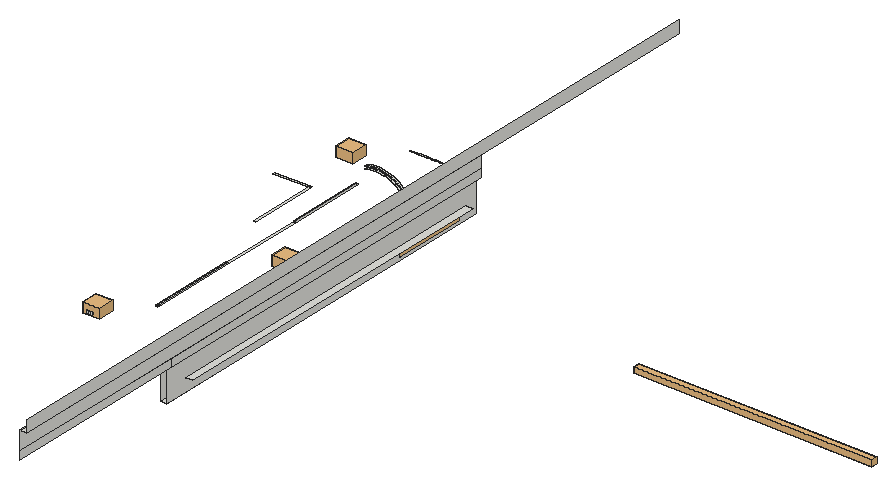
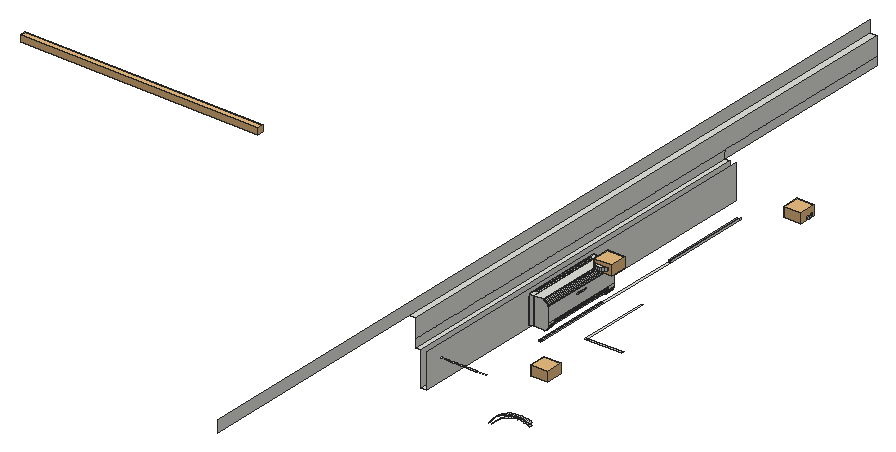
# SketchUp Ruby script. Lengths in inches.
U = 1.inch
M = Sketchup.active_model
def pt(a) = Geom::Point3d.new(a.map { |v| v * U })
def face(e, loops, mat)
  f = e.add_face(loops[0].map { |a| pt(a) })
  loops[1..].each { |l| e.add_face(l.map { |a| pt(a) }).erase! }
  f.material = f.back_material = mat if mat
  f
end
# faces: each face lists its corners as indices into pts; further lists are holes
def faces(e, pts, list, mat = nil) = list.each { |f| face(e, (f[0].is_a?(Array) ? f : [f]).map { |l| l.map { |i| pts[i] } }, mat) }
# xy, xz, yz: faces in a plane at the given z, y or x. An outline is a flat list of corners, or four numbers for a rectangle; further outlines are holes
def ring(l) = l.size == 4 ? [[l[0], l[1]], [l[2], l[1]], [l[2], l[3]], [l[0], l[3]]] : l.each_slice(2).to_a
def flat(e, list, mat, &to3) = list.each { |f| face(e, (f[0].is_a?(Array) ? f : [f]).map { |l| ring(l).map { |u, v| to3.(u, v) } }, mat) }
def xy(e, z, list, mat = nil) = flat(e, list, mat) { |x, y| [x, y, z] }
def xz(e, y, list, mat = nil) = flat(e, list, mat) { |x, z| [x, y, z] }
def yz(e, x, list, mat = nil) = flat(e, list, mat) { |y, z| [x, y, z] }
def lines(e, pts, list) = list.each { |a, b| e.add_line(pt(pts[a]), pt(pts[b])) }
# prism: a flat outline (further loops are holes) pulled along v
def prism(e, loops, v, mat = nil)
  f = face(e, loops, mat); d = Geom::Vector3d.new(v.map { |x| x * U })
  f.pushpull(f.normal.samedirection?(d) ? d.length : -d.length)
end
def box(e, o, s, mat = nil) = prism(e, [[o, [o[0] + s[0], o[1], o[2]], [o[0] + s[0], o[1] + s[1], o[2]], [o[0], o[1] + s[1], o[2]]]], [0, 0, s[2]], mat)
def at(x, y, z, deg = 0) = Geom::Transformation.translation(pt([x, y, z])) * Geom::Transformation.rotation(ORIGIN, Z_AXIS, deg.degrees)
def axes(o, x, y, z) = Geom::Transformation.new([*x, 0, *y, 0, *z, 0, *pt(o).to_a, 1])
def part(name) = M.definitions.add(name)
# library, detail: a bought-in or finely detailed component or shape, given as its bounding box
def library(name, o, s) = part(name).tap { |d| box(d.entities, o, s) }
def detail(e, o, s) = box(e.add_group.entities, o, s)
def put(e, d, t, mat = nil) = e.add_instance(d, t).tap { |i| i.material = mat if mat }
def group(e, t, mat = nil) = e.add_group.tap { |g| g.transformation = t; g.material = mat if mat }.entities
root = M.entities
M.materials.add("[Color_004]").color = [142, 142, 142]
M.materials.add("[Color_007]").color = [58, 58, 58]
M.materials.add("[Color_C12]").color = [153, 91, 30]
c1 = library("10 (1)",[26.65,-5.45,122.92],[1.37,1.38,0.36])
c2 = library("Group\#18",[-88.79,21.34,-41.3125],[0.99,6.53,4.87])
c3 = library("Group\#15",[-88.79,0.67,-41.3125],[0.99,6.14,4.87])
c4 = library("Group\#19",[-80.46,-65.36,-92.6],[1.38,3.58,3.59])
c5 = library("Group\#9",[-80.34,-149.03,-93.91],[1.18,2.79,3])
c6 = library("Group\#8",[-80.34,-139.83,-93.89],[1.18,2.84,2.98])
c7 = library("Component\#44",[-0.76,-0.76,-71.54],[3.88,3.88,152.54])
xy(root,91.83,[[286.12,96.9375,289,294.91]])
xy(root,100.73,[[291.63,105.89,295.1875,285.58]])
xy(root,109.39,[[289,96.9375,291.63,294.91],[255.63,131.9375,256.63,132.9375],[255.63,176.87,256.63,220.26],[242.63,211.08,243.63,245.91],[224.48,245.91,242.63,246.91],
  [242.63,245.91,243.63,246.91],[255.93,294.47,260.26,294.91],[260.79,294.47,264.44,294.91],[264.79,294.47,266.48,294.91],[266.83,294.47,268.52,294.91],
  [268.86,294.47,270.55,294.91],[270.9,294.47,272.59,294.91],[272.94,294.47,274.63,294.91],[274.98,294.47,276.67,294.91],[277.02,294.47,278.7,294.91]])
xy(root,109.96,[[255.63,220.26,256.63,258.91],[255.63,258.91,256.63,259.91]])
xy(root,110.08,[[255.63,132.9375,256.63,176.87]])
xy(root,110.77,[[238.63,109.9375,237.6,110.07,236.63,110.47,235.8,111.11,235.17,111.9375,234.77,112.9,234.63,113.9375,234.77,114.97,235.17,115.9375,235.8,116.77,236.63,117.4,237.6,117.8,238.63,117.9375,239.67,117.8,240.63,117.4,241.46,116.77,242.09,115.9375,242.49,114.97,242.63,113.9375,242.49,112.9,242.09,111.9375,241.46,111.11,240.63,110.47,239.67,110.07],[274.63,191.92,273.6,192.06,272.63,192.46,271.8,193.09,271.17,193.92,270.77,194.89,270.63,195.92,270.77,196.96,271.17,197.92,271.8,198.75,272.63,199.39,273.6,199.79,274.63,199.92,275.67,199.79,276.63,199.39,277.46,198.75,278.09,197.92,278.49,196.96,278.63,195.92,278.49,194.89,278.09,193.92,277.46,193.09,276.63,192.46,275.67,192.06],[238.63,273.91,237.6,274.04,236.63,274.44,235.8,275.08,235.17,275.91,234.77,276.87,234.63,277.91,234.77,278.94,235.17,279.91,235.8,280.73,236.63,281.37,237.6,281.77,238.63,281.91,239.67,281.77,240.63,281.37,241.46,280.73,242.09,279.91,242.49,278.94,242.63,277.91,242.49,276.87,242.09,275.91,241.46,275.08,240.63,274.44,239.67,274.04]])
xy(root,123.125,[[291.63,0,295.1875,294.91]])
xz(root,132.9375,[[255.63,109.39,256.63,110.08]])
xz(root,176.87,[[255.63,109.39,256.63,110.08]])
xz(root,220.26,[[255.63,109.39,256.63,109.96]])
xz(root,259.91,[[255.63,109.39,256.63,109.96]])
yz(root,255.63,[[131.9375,109.39,132.9375,110.08],[132.9375,109.39,176.87,110.08],[220.26,109.39,258.91,109.96]])
yz(root,256.63,[[132.9375,109.39,176.87,110.08],[220.26,109.39,258.91,109.96],[258.91,109.39,259.91,109.96]])
yz(root,286.12,[[96.9375,91.83,294.91,109.39]])
yz(root,289,[[96.9375,91.83,294.91,109.39]])
yz(root,291.63,[[0,109.39,96.9375,113.39],[96.9375,109.39,294.91,113.39],[0,113.39,294.91,123.125]])
yz(root,295.1875,[[0,123.125,417.6875,129.125]])
p = [[252.54,293.53,88.43],[252.54,294.66,88.43],[252.91,294.66,87.83],[252.91,293.53,87.83],[254.51,294.91,87.98],[254.05,294.91,88.63],
  [254.05,293.53,88.63],[254.51,293.53,87.98],[249.64,294.91,91.08],[249.79,294.91,90.9375],[249.79,294.66,90.9375],[249.64,293.53,91.08],
  [249.64,294.66,91.08],[253.55,294.91,89.26],[253.55,293.53,89.26],[253.03,294.91,89.87],[253.03,293.53,89.87],[252.48,294.91,90.45],
  [252.48,293.53,90.45],[251.91,294.91,91.01],[251.91,293.53,91.01],[251.3125,294.91,91.55],[251.3125,293.53,91.55],[248.89,293.53,91.75],
  [248.89,294.66,91.75],[250.69,294.91,92.05],[250.69,293.53,92.05],[246.67,294.91,92.83],[246.8,294.91,92.76],[246.8,294.66,92.76],
  [246.67,293.53,92.83],[246.67,294.66,92.83],[250.06,294.91,92.53],[250.06,293.53,92.53],[249.4,294.91,92.99],[249.4,293.53,92.99],
  [244.44,293.53,93.9],[244.44,294.66,93.9],[248.72,294.91,93.41],[248.72,293.53,93.41],[248.02,294.91,93.8],[248.02,293.53,93.8],
  [233.34,294.91,93.47],[233.56,294.91,93.57],[233.56,294.66,93.57],[234.67,294.66,94.0625],[234.67,293.53,94.0625],[233.34,293.53,93.47],
  [233.34,294.66,93.47],[247.31,294.91,94.16],[247.31,293.53,94.16],[243.24,294.91,94.09],[243.31,294.91,94.08],[243.31,294.66,94.08],
  [243.24,293.53,94.09],[243.24,294.66,94.09],[236.33,294.66,94.28],[236.33,293.53,94.28],[239.57,294.91,94.69],[239.66,294.91,94.68],
  [239.66,294.66,94.68],[239.57,293.53,94.69],[239.57,294.41,94.69],[246.58,294.91,94.5],[246.58,293.53,94.5],[236.33,294.91,94.28],
  [236.47,294.91,94.29],[236.47,294.41,94.29],[245.84,294.91,94.8],[245.84,293.53,94.8],[245.08,294.91,95.0625],[245.08,293.53,95.0625],
  [234.05,294.91,95.24],[233.29,294.91,95],[233.29,293.53,95],[234.05,293.53,95.24],[244.32,294.91,95.3],[244.32,293.53,95.3],
  [234.83,294.91,95.45],[234.83,293.53,95.45],[243.54,294.91,95.5],[243.54,293.53,95.5],[235.61,294.91,95.63],[235.61,293.53,95.63],
  [242.76,294.91,95.67],[242.76,293.53,95.67],[236.39,294.91,95.77],[236.39,293.53,95.77],[241.97,294.91,95.8],[241.97,293.53,95.8],
  [237.1875,294.91,95.88],[237.1875,293.53,95.88],[241.18,294.91,95.9],[241.18,293.53,95.9],[237.98,294.91,95.95],[237.98,293.53,95.95],
  [240.38,294.91,95.97],[240.38,293.53,95.97],[238.78,294.91,95.99],[238.78,293.53,95.99],[239.58,294.91,96],[239.58,293.53,96],
  [238.63,109.9375,109.39],[237.6,110.07,109.39],[237.6,110.07,110.77],[238.63,109.9375,110.77],[239.67,110.07,109.39],[239.67,110.07,110.77],
  [236.63,110.47,109.39],[236.63,110.47,110.77],[240.63,110.47,109.39],[240.63,110.47,110.77],[235.8,111.11,109.39],[235.8,111.11,110.77],
  [241.46,111.11,109.39],[241.46,111.11,110.77],[235.17,111.9375,109.39],[235.17,111.9375,110.77],[242.09,111.9375,109.39],[242.09,111.9375,110.77],
  [234.77,112.9,109.39],[234.77,112.9,110.77],[242.49,112.9,109.39],[242.49,112.9,110.77],[234.63,113.9375,109.39],[234.63,113.9375,110.77],
  [242.63,113.9375,109.39],[242.63,113.9375,110.77],[234.77,114.97,109.39],[234.77,114.97,110.77],[242.49,114.97,109.39],[242.49,114.97,110.77],
  [235.17,115.9375,109.39],[235.17,115.9375,110.77],[242.09,115.9375,109.39],[242.09,115.9375,110.77],[235.8,116.77,109.39],[235.8,116.77,110.77],
  [241.46,116.77,109.39],[241.46,116.77,110.77],[236.63,117.4,109.39],[236.63,117.4,110.77],[240.63,117.4,109.39],[240.63,117.4,110.77],
  [237.6,117.8,109.39],[237.6,117.8,110.77],[239.67,117.8,109.39],[239.67,117.8,110.77],[238.63,117.9375,109.39],[238.63,117.9375,110.77],
  [274.63,191.92,109.39],[273.6,192.06,109.39],[273.6,192.06,110.77],[274.63,191.92,110.77],[275.67,192.06,109.39],[275.67,192.06,110.77],
  [272.63,192.46,109.39],[272.63,192.46,110.77],[276.63,192.46,109.39],[276.63,192.46,110.77],[271.8,193.09,109.39],[271.8,193.09,110.77],
  [277.46,193.09,109.39],[277.46,193.09,110.77],[271.17,193.92,109.39],[271.17,193.92,110.77],[278.09,193.92,109.39],[278.09,193.92,110.77],
  [270.77,194.89,109.39],[270.77,194.89,110.77],[278.49,194.89,109.39],[278.49,194.89,110.77],[270.63,195.92,109.39],[270.63,195.92,110.77],
  [278.63,195.92,109.39],[278.63,195.92,110.77],[270.77,196.96,109.39],[270.77,196.96,110.77],[278.49,196.96,109.39],[278.49,196.96,110.77],
  [271.17,197.92,109.39],[271.17,197.92,110.77],[278.09,197.92,109.39],[278.09,197.92,110.77],[271.8,198.75,109.39],[271.8,198.75,110.77],
  [277.46,198.75,109.39],[277.46,198.75,110.77],[272.63,199.39,109.39],[272.63,199.39,110.77],[276.63,199.39,109.39],[276.63,199.39,110.77],
  [273.6,199.79,109.39],[273.6,199.79,110.77],[275.67,199.79,109.39],[275.67,199.79,110.77],[274.63,199.92,109.39],[274.63,199.92,110.77],
  [238.63,273.91,109.39],[237.6,274.04,109.39],[237.6,274.04,110.77],[238.63,273.91,110.77],[239.67,274.04,109.39],[239.67,274.04,110.77],
  [236.63,274.44,109.39],[236.63,274.44,110.77],[240.63,274.44,109.39],[240.63,274.44,110.77],[235.8,275.08,109.39],[235.8,275.08,110.77],
  [241.46,275.08,109.39],[241.46,275.08,110.77],[235.17,275.91,109.39],[235.17,275.91,110.77],[242.09,275.91,109.39],[242.09,275.91,110.77],
  [234.77,276.87,109.39],[234.77,276.87,110.77],[242.49,276.87,109.39],[242.49,276.87,110.77],[234.63,277.91,109.39],[234.63,277.91,110.77],
  [242.63,277.91,109.39],[242.63,277.91,110.77],[234.77,278.94,109.39],[234.77,278.94,110.77],[242.49,278.94,109.39],[242.49,278.94,110.77],
  [235.17,279.91,109.39],[235.17,279.91,110.77],[242.09,279.91,109.39],[242.09,279.91,110.77],[235.8,280.73,109.39],[235.8,280.73,110.77],
  [241.46,280.73,109.39],[241.46,280.73,110.77],[236.63,281.37,109.39],[236.63,281.37,110.77],[240.63,281.37,109.39],[240.63,281.37,110.77],
  [237.6,281.77,109.39],[237.6,281.77,110.77],[239.67,281.77,109.39],[239.67,281.77,110.77],[238.63,281.91,109.39],[238.63,281.91,110.77]]
faces(root,p,[[0,1,2,3],[4,5,6,7],[8,9,10,1,0,11,12],[5,13,14,6],[13,15,16,14],[15,17,18,16],[17,19,20,18],[19,21,22,20],
  [23,24,12,11],[21,25,26,22],[27,28,29,24,23,30,31],[25,32,33,26],[32,34,35,33],[36,37,31,30],[34,38,39,35],[38,40,41,39],
  [42,43,44,45,46,47,48],[40,49,50,41],[51,52,53,37,36,54,55],[46,45,56,57],[58,59,60,55,54,61,62],[49,63,64,50],[65,66,67,62,61,57,56],[63,68,69,64],
  [68,70,71,69],[72,73,74,75],[70,76,77,71],[78,72,75,79],[76,80,81,77],[82,78,79,83],[80,84,85,81],[86,82,83,87],
  [84,88,89,85],[90,86,87,91],[88,92,93,89],[94,90,91,95],[92,96,97,93],[98,94,95,99],[100,98,99,101],[96,100,101,97],
  [102,103,104,105],[106,102,105,107],[103,108,109,104],[110,106,107,111],[108,112,113,109],[114,110,111,115],[112,116,117,113],[118,114,115,119],
  [116,120,121,117],[122,118,119,123],[120,124,125,121],[126,122,123,127],[124,128,129,125],[130,126,127,131],[128,132,133,129],[134,130,131,135],
  [132,136,137,133],[138,134,135,139],[136,140,141,137],[142,138,139,143],[140,144,145,141],[146,142,143,147],[144,148,149,145],[148,146,147,149],
  [150,151,152,153],[154,150,153,155],[151,156,157,152],[158,154,155,159],[156,160,161,157],[162,158,159,163],[160,164,165,161],[166,162,163,167],
  [164,168,169,165],[170,166,167,171],[168,172,173,169],[174,170,171,175],[172,176,177,173],[178,174,175,179],[176,180,181,177],[182,178,179,183],
  [180,184,185,181],[186,182,183,187],[184,188,189,185],[190,186,187,191],[188,192,193,189],[194,190,191,195],[192,196,197,193],[196,194,195,197],
  [198,199,200,201],[202,198,201,203],[199,204,205,200],[206,202,203,207],[204,208,209,205],[210,206,207,211],[208,212,213,209],[214,210,211,215],
  [212,216,217,213],[218,214,215,219],[216,220,221,217],[222,218,219,223],[220,224,225,221],[226,222,223,227],[224,228,229,225],[230,226,227,231],
  [228,232,233,229],[234,230,231,235],[232,236,237,233],[238,234,235,239],[236,240,241,237],[242,238,239,243],[240,244,245,241],[244,242,243,245]])
put(root,c1,axes([61.11,307.48,-1589.04],[6.49609,0,0],[0,6.19526,0],[0,0,13.8072]))
put(root,c1,axes([62.02,144.11,-1588.37],[6.49609,0,0],[0,6.19526,0],[0,0,13.8072]))
put(root,c1,axes([96.18,222.92,-1589.66],[6.49609,0,0],[0,6.19526,0],[0,0,13.8072]))
g1 = group(root,at(286.12,208.66,107.43))
detail(g1,[-10.16,1.62,-4.73],[0.11,0.74,0.56])
g2 = group(root,at(286.12,208.66,107.43),"[Color_004]")
prism(g2,[[[-10.05,-1.59,-4.73],[-10.05,-1.41,-4.73],[-10.05,-1.55,-4.17],[-10.05,-1.79,-4.17],[-10.05,-1.91,-4.55],[-10.05,-2.04,-4.17],[-10.05,-2.26,-4.17],[-10.05,-2.41,-4.73],[-10.05,-2.23,-4.73],[-10.05,-2.13,-4.36],[-10.05,-2.01,-4.73],[-10.05,-1.82,-4.73],[-10.05,-1.69,-4.34]]],[-0.11,0,0],"[Color_004]")
put(root,c2,axes([286.12,208.66,107.43],[0.11448,0,0],[0,0.11448,0],[0,0,0.11448]))
put(root,c3,axes([286.12,208.66,107.43],[0.11448,0,0],[0,0.11448,0],[0,0,0.11448]))
g3 = group(root,at(286.12,208.66,107.43))
detail(g3,[-10.16,-3.17,-4.73],[0.11,0.72,0.56])
g4 = group(root,at(286.12,208.66,107.43))
prism(g4,[[[-10.05,0.02,-4.3],[-10.05,0.02,-4.17],[-10.05,-0.6,-4.17],[-10.05,-0.6,-4.3],[-10.05,-0.39,-4.3],[-10.05,-0.39,-4.73],[-10.05,-0.19,-4.73],[-10.05,-0.19,-4.3]]],[-0.11,0,0],"[Color_004]")
g5 = group(root,at(286.12,208.66,107.43))
prism(g5,[[[-10.05,1.44,-4.73],[-10.05,1.65,-4.73],[-10.05,1.34,-4.2],[-10.05,1.34,-4.19],[-10.05,1.33,-4.18],[-10.05,1.31,-4.18],[-10.05,1.3,-4.17],[-10.05,1.29,-4.17],[-10.05,1.15,-4.17],[-10.05,1.14,-4.17],[-10.05,1.125,-4.18],[-10.05,1.12,-4.18],[-10.05,1.11,-4.19],[-10.05,1.1,-4.2],[-10.05,0.8,-4.73],[-10.05,1,-4.73],[-10.05,1.07,-4.61],[-10.05,1.37,-4.61]],[[-10.05,1.32,-4.52],[-10.05,1.12,-4.52],[-10.05,1.22,-4.35]]],[-0.11,0,0],"[Color_004]")
g6 = group(root,at(286.12,208.66,107.43))
detail(g6,[-10.16,-1.36,-4.73],[0.11,0.71,0.56])
g7 = group(root,at(286.12,208.66,107.43))
prism(g7,[[[-10.05,-0.91,-4.52],[-10.05,-0.85,-4.39],[-10.05,-1.27,-4.39],[-10.05,-1.36,-4.52]]],[-0.11,0,0],"[Color_004]")
put(root,c4,axes([286.02,208.66,107.43],[0.11448,0,0],[0,0.11448,0],[0,0,0.11448]))
put(root,c5,axes([286.04,208.66,107.43],[0.11448,0,0],[0,0.11448,0],[0,0,0.11448]))
g8 = group(root,at(286.04,208.66,107.43))
detail(g8,[-9.2,-17.18,-10.75],[0.14,0.08,0.08])
g9 = group(root,at(286.04,208.66,107.43))
detail(g9,[-9.2,-16.3125,-10.75],[0.14,0.28,0.46])
put(root,c6,axes([286.04,208.66,107.43],[0.11448,0,0],[0,0.11448,0],[0,0,0.11448]))
g10 = group(root,at(286.04,208.66,107.43),"[Color_004]")
prism(g10,[[[-9.2,-16.69,-10.41],[-9.2,-16.57,-10.63],[-9.2,-16.52,-10.41],[-9.2,-16.45,-10.41],[-9.2,-16.52,-10.74],[-9.2,-16.6,-10.74],[-9.2,-16.78,-10.41]]],[0.14,0,0],"[Color_004]")
g11 = group(root,at(286.04,208.66,107.43))
prism(g11,[[[-9.2,-16.38,-10.74],[-9.2,-16.43,-10.41],[-9.2,-16.36,-10.41],[-9.2,-16.3,-10.74]]],[0.14,0,0],"[Color_004]")
g12 = group(root,at(286.04,208.66,107.43))
prism(g12,[[[-9.2,-17.17,-10.29],[-9.2,-17.11,-10.63],[-9.2,-17.1875,-10.63],[-9.2,-17.24,-10.29]]],[0.14,0,0],"[Color_004]")
g13 = group(root,at(286.04,208.66,107.43))
detail(g13,[-9.2,-16.46,-10.375],[0.14,0.09,0.09])
g14 = group(root,at(286.12,208.66,107.43))
prism(g14,[[[-10.05,20.75,-9.92],[-10.05,20.75,-2.7],[-10.02,20.75,-2.28],[-9.92,20.75,-1.87],[-9.76,20.75,-1.48],[-9.53,20.75,-1.11],[-9.26,20.75,-0.79],[-8.9375,20.75,-0.52],[-8.57,20.75,-0.29],[-8.18,20.75,-0.13],[-7.77,20.75,-0.03],[-7.35,20.75,0],[-7.35,20.75,-0.14],[-7.75,20.75,-0.17],[-8.14,20.75,-0.26],[-8.51,20.75,-0.42],[-8.86,20.75,-0.625],[-9.16,20.75,-0.89],[-9.42,20.75,-1.19],[-9.64,20.75,-1.54],[-9.79,20.75,-1.91],[-9.88,20.75,-2.3],[-9.92,20.75,-2.7],[-9.92,20.75,-9.92]]],[0,-41.5,0])
g15 = group(root,at(286.12,208.66,107.43))
xy(g15,-13.71,[[-7.26,-17.58,-4.78,17.58]])
xy(g15,-11.54,[[-9.43,-17.58,-9.11,-10.08],[-9.43,-9.81,-9.11,5.21],[-9.43,5.48,-9.11,17.58]])
xy(g15,-10.97,[[-9.11,-17.58,-4.78,-17.58,-4.78,17.58,-9.11,17.58,-9.11,5.48,-9.43,5.48,-9.43,5.21,-9.11,5.21,-9.11,-9.81,-9.43,-9.81,-9.43,-10.08,-9.11,-10.08]])
xz(g15,-17.58,[[-7.26,-13.71,-4.78,-13.71,-4.78,-10.97,-9.11,-10.97,-9.11,-11.54,-9.43,-11.54,-9.42,-11.59,-9.4,-11.88,-9.32,-12.21,-9.19,-12.52,-9.01,-12.8125,-8.79,-13.07,-8.54,-13.29,-8.25,-13.47,-7.93,-13.6,-7.6,-13.68]])
xz(g15,-10.08,[[-9.43,-11.54,-9.11,-10.97]])
xz(g15,-9.81,[[-9.43,-11.54,-9.11,-10.97]])
xz(g15,5.21,[[-9.43,-11.54,-9.11,-10.97]])
xz(g15,5.48,[[-9.43,-11.54,-9.11,-10.97]])
xz(g15,17.58,[[-7.26,-13.71,-7.6,-13.68,-7.93,-13.6,-8.25,-13.47,-8.54,-13.29,-8.79,-13.07,-9.01,-12.8125,-9.19,-12.52,-9.32,-12.21,-9.4,-11.88,-9.42,-11.59,-9.43,-11.54,-9.11,-11.54,-9.11,-10.97,-4.78,-10.97,-4.78,-13.71]])
yz(g15,-9.43,[[-10.08,-11.54,-9.81,-10.97],[5.21,-11.54,5.48,-10.97]])
yz(g15,-9.11,[[-17.58,-11.54,-10.08,-10.97],[-9.81,-11.54,5.21,-10.97],[5.48,-11.54,17.58,-10.97]],"[Color_007]")
yz(g15,-4.78,[[-17.58,-13.71,17.58,-10.97]])
p = [[-7.93,-17.58,-13.6],[-7.93,17.58,-13.6],[-7.6,17.58,-13.68],[-7.6,-17.58,-13.68],[-7.26,17.58,-13.71],[-7.26,-17.58,-13.71],
  [-8.25,17.58,-13.47],[-8.25,-17.58,-13.47],[-8.54,-17.58,-13.29],[-8.54,17.58,-13.29],[-8.79,-17.58,-13.07],[-8.79,17.58,-13.07],
  [-9.01,-17.58,-12.8125],[-9.01,17.58,-12.8125],[-9.19,-17.58,-12.52],[-9.19,17.58,-12.52],[-9.32,17.58,-12.21],[-9.32,-17.58,-12.21],
  [-9.4,-17.58,-11.88],[-9.4,17.58,-11.88],[-9.42,-17.58,-11.59],[-9.42,-10.08,-11.59],[-9.42,-9.81,-11.59],[-9.42,5.21,-11.59],
  [-9.42,5.48,-11.59],[-9.42,17.58,-11.59],[-9.43,17.58,-11.54],[-9.43,-17.58,-11.54],[-9.43,-10.08,-11.54],[-9.43,-9.81,-11.54],
  [-9.43,5.21,-11.54],[-9.43,5.48,-11.54]]
faces(g15,p,[[0,1,2,3],[4,5,3,2],[6,1,0,7],[6,7,8,9],[10,11,9,8],[11,10,12,13],[14,15,13,12],[16,15,14,17],
  [16,17,18,19],[18,20,21,22,23,24,25,19]])
faces(g15,p,[[26,25,24,23,22,21,20,27,28,29,30,31]],"[Color_C12]")
g16 = group(root,at(286.12,208.66,107.43))
xy(g16,-14.11,[[-7.35,-20.77,-2.25,-17.58],[-7.35,17.58,-2.25,20.77]])
xy(g16,-10.97,[[-9.15,-17.58,-2.25,17.58]])
xy(g16,-10.75,[[-9.15,-3.86,-9.01,3.86]])
xy(g16,-10.04,[[-9.15,-3.86,-9.01,3.86]])
xy(g16,-9.92,[[-10.05,-20.77,-9.92,-17.58],[-9.92,-17.58,-9.15,17.58],[-10.05,17.58,-9.92,20.77]])
xy(g16,0,[[-7.35,-20.77,-2.25,20.77]])
xz(g16,-20.77,[[-7.35,-14.11,-2.25,-14.11,-2.25,0,-7.35,0,-7.35,-0.14,-7.75,-0.17,-8.14,-0.26,-8.51,-0.42,-8.86,-0.625,-9.16,-0.89,-9.42,-1.19,-9.64,-1.54,-9.79,-1.91,-9.88,-2.3,-9.92,-2.7,-9.92,-9.92,-10.05,-9.92,-10.05,-11.4,-10.02,-11.83,-9.92,-12.24,-9.76,-12.63,-9.53,-12.99,-9.26,-13.32,-8.9375,-13.59,-8.57,-13.8125,-8.18,-13.97,-7.77,-14.07]])
xz(g16,-17.58,[[-7.35,-14.11,-7.77,-14.07,-8.18,-13.97,-8.57,-13.8125,-8.9375,-13.59,-9.26,-13.32,-9.53,-12.99,-9.76,-12.63,-9.92,-12.24,-10.02,-11.83,-10.05,-11.4,-10.05,-9.92,-9.15,-9.92,-9.15,-10.97,-2.25,-10.97,-2.25,-14.11]])
xz(g16,-3.86,[[-9.15,-10.75,-9.01,-10.04]])
xz(g16,3.86,[[-9.15,-10.75,-9.01,-10.04]])
xz(g16,17.58,[[-7.35,-14.11,-2.25,-14.11,-2.25,-10.97,-9.15,-10.97,-9.15,-9.92,-10.05,-9.92,-10.05,-11.4,-10.02,-11.83,-9.92,-12.24,-9.76,-12.63,-9.53,-12.99,-9.26,-13.32,-8.9375,-13.59,-8.57,-13.8125,-8.18,-13.97,-7.77,-14.07]])
xz(g16,20.77,[[-7.35,-14.11,-7.77,-14.07,-8.18,-13.97,-8.57,-13.8125,-8.9375,-13.59,-9.26,-13.32,-9.53,-12.99,-9.76,-12.63,-9.92,-12.24,-10.02,-11.83,-10.05,-11.4,-10.05,-9.92,-9.92,-9.92,-9.92,-2.7,-9.88,-2.3,-9.79,-1.91,-9.64,-1.54,-9.42,-1.19,-9.16,-0.89,-8.86,-0.625,-8.51,-0.42,-8.14,-0.26,-7.75,-0.17,-7.35,-0.14,-7.35,0,-2.25,0,-2.25,-14.11]])
yz(g16,-10.05,[[-20.77,-11.4,-17.58,-9.92],[17.58,-11.4,20.77,-9.92]])
yz(g16,-9.92,[[-20.77,-9.92,20.77,-2.7]])
yz(g16,-9.15,[[[-17.58,-10.97,17.58,-9.92],[-3.86,-10.75,3.86,-10.04]]])
yz(g16,-9.01,[[-3.86,-10.75,3.86,-10.04]],"[Color_007]")
yz(g16,-7.35,[[-20.77,-0.14,20.77,0]])
yz(g16,-2.25,[[-20.77,-14.11,-17.58,-14.11,-17.58,-10.97,17.58,-10.97,17.58,-14.11,20.77,-14.11,20.77,0,-20.77,0]])
p = [[-8.18,-20.77,-13.97],[-8.18,-17.58,-13.97],[-7.77,-17.58,-14.07],[-7.77,-20.77,-14.07],[-7.35,-17.58,-14.11],[-7.35,-20.77,-14.11],
  [-8.18,17.58,-13.97],[-8.18,20.77,-13.97],[-7.77,20.77,-14.07],[-7.77,17.58,-14.07],[-7.35,20.77,-14.11],[-7.35,17.58,-14.11],
  [-8.57,-17.58,-13.8125],[-8.57,-20.77,-13.8125],[-8.57,17.58,-13.8125],[-8.57,20.77,-13.8125],[-8.9375,-20.77,-13.59],[-8.9375,-17.58,-13.59],
  [-8.9375,17.58,-13.59],[-8.9375,20.77,-13.59],[-9.26,-20.77,-13.32],[-9.26,-17.58,-13.32],[-9.26,17.58,-13.32],[-9.26,20.77,-13.32],
  [-9.53,-20.77,-12.99],[-9.53,-17.58,-12.99],[-9.53,17.58,-12.99],[-9.53,20.77,-12.99],[-9.76,-20.77,-12.63],[-9.76,-17.58,-12.63],
  [-9.76,17.58,-12.63],[-9.76,20.77,-12.63],[-9.92,-17.58,-12.24],[-9.92,-20.77,-12.24],[-9.92,17.58,-12.24],[-9.92,20.77,-12.24],
  [-10.02,-20.77,-11.83],[-10.02,-17.58,-11.83],[-10.02,17.58,-11.83],[-10.02,20.77,-11.83],[-10.05,-20.77,-11.4],[-10.05,-17.58,-11.4],
  [-10.05,17.58,-11.4],[-10.05,20.77,-11.4],[-9.92,20.77,-2.7],[-9.92,-20.77,-2.7],[-9.88,-20.77,-2.3],[-9.88,20.77,-2.3],
  [-9.79,-20.77,-1.91],[-9.79,20.77,-1.91],[-9.64,20.77,-1.54],[-9.64,-20.77,-1.54],[-9.42,-20.77,-1.19],[-9.42,20.77,-1.19],
  [-9.16,-20.77,-0.89],[-9.16,20.77,-0.89],[-8.86,-20.77,-0.625],[-8.86,20.77,-0.625],[-8.51,-20.77,-0.42],[-8.51,20.77,-0.42],
  [-8.14,20.77,-0.26],[-8.14,-20.77,-0.26],[-7.75,-20.77,-0.17],[-7.75,20.77,-0.17],[-7.35,-20.77,-0.14],[-7.35,20.77,-0.14]]
faces(g16,p,[[0,1,2,3],[4,5,3,2],[6,7,8,9],[10,11,9,8],[12,1,0,13],[6,14,15,7],[12,13,16,17],[15,14,18,19],
  [20,21,17,16],[22,23,19,18],[21,20,24,25],[23,22,26,27],[28,29,25,24],[30,31,27,26],[32,29,28,33],[30,34,35,31],
  [32,33,36,37],[35,34,38,39],[40,41,37,36],[42,43,39,38],[44,45,46,47],[48,49,47,46],[50,49,48,51],[50,51,52,53],
  [54,55,53,52],[55,54,56,57],[58,59,57,56],[60,59,58,61],[60,61,62,63],[64,65,63,62]])
g17 = group(root,at(286.12,208.66,107.43))
xy(g17,-14.11,[[-2.25,-20.77,0,20.77]])
xy(g17,-2.51,[[-1.22,-17.36,-0.95,-13.22],[-0.84,-17.36,-0.57,-13.22],[-0.46,-17.36,-0.1875,-13.22],[-1.22,-12.99,-0.95,-8.85],[-0.84,-12.99,-0.57,-8.85],
  [-0.46,-12.99,-0.1875,-8.85],[-1.22,-8.625,-0.95,-4.48],[-0.84,-8.625,-0.57,-4.48],[-0.46,-8.625,-0.1875,-4.48],[-1.22,-4.26,-0.95,-0.11],
  [-0.84,-4.26,-0.57,-0.11],[-0.46,-4.26,-0.1875,-0.11],[-1.22,0.11,-0.95,4.26],[-0.84,0.11,-0.57,4.26],[-0.46,0.11,-0.1875,4.26],
  [-1.22,4.48,-0.95,8.625],[-0.84,4.48,-0.57,8.625],[-0.46,4.48,-0.1875,8.625],[-1.22,8.85,-0.95,12.99],[-0.84,8.85,-0.57,12.99],
  [-0.46,8.85,-0.1875,12.99],[-1.22,13.22,-0.95,17.36],[-0.84,13.22,-0.57,17.36],[-0.46,13.22,-0.1875,17.36]])
xy(g17,0,[[[-2.25,-20.77,0,20.77],[-1.22,4.48,-1.22,12.99,-0.95,12.99,-0.95,8.85,-1.22,8.85,-1.22,8.625,-0.95,8.625,-0.95,4.48],[-0.46,4.48,-0.46,8.625,-0.1875,8.625,-0.1875,8.85,-0.46,8.85,-0.46,12.99,-0.1875,12.99,-0.1875,4.48],[-0.84,13.22,-0.57,17.36],[-0.46,13.22,-0.1875,17.36],[-1.22,13.22,-0.95,17.36],[-1.22,-17.36,-0.95,-13.22],[-0.46,-17.36,-0.1875,-13.22],[-0.84,-17.36,-0.57,-13.22],[-0.84,4.48,-0.57,8.625],[-0.46,-8.625,-0.1875,-4.48],[-0.84,-8.625,-0.57,-4.48],[-1.22,-8.625,-0.95,-4.48],[-0.84,8.85,-0.57,12.99],[-0.84,0.11,-0.57,4.26],[-0.46,0.11,-0.1875,4.26],[-1.22,0.11,-0.95,4.26],[-0.46,-12.99,-0.1875,-8.85],[-1.22,-12.99,-0.95,-8.85],[-1.22,-4.26,-0.95,-0.11],[-0.84,-4.26,-0.57,-0.11],[-0.46,-4.26,-0.1875,-0.11],[-0.84,-12.99,-0.57,-8.85]]])
xz(g17,-20.77,[[-2.25,-14.11,0,0]])
xz(g17,-17.36,[[-1.22,-2.51,-0.95,0],[-0.84,-2.51,-0.57,0],[-0.46,-2.51,-0.1875,0]])
xz(g17,-13.22,[[-1.22,-2.51,-0.95,0],[-0.84,-2.51,-0.57,0],[-0.46,-2.51,-0.1875,0]])
xz(g17,-12.99,[[-1.22,-2.51,-0.95,0],[-0.84,-2.51,-0.57,0],[-0.46,-2.51,-0.1875,0]])
xz(g17,-8.85,[[-1.22,-2.51,-0.95,0],[-0.84,-2.51,-0.57,0],[-0.46,-2.51,-0.1875,0]])
xz(g17,-8.625,[[-1.22,-2.51,-0.95,0],[-0.84,-2.51,-0.57,0],[-0.46,-2.51,-0.1875,0]])
xz(g17,-4.48,[[-1.22,-2.51,-0.95,0],[-0.84,-2.51,-0.57,0],[-0.46,-2.51,-0.1875,0]])
xz(g17,-4.26,[[-1.22,-2.51,-0.95,0],[-0.84,-2.51,-0.57,0],[-0.46,-2.51,-0.1875,0]])
xz(g17,-0.11,[[-1.22,-2.51,-0.95,0],[-0.84,-2.51,-0.57,0],[-0.46,-2.51,-0.1875,0]])
xz(g17,0.11,[[-1.22,-2.51,-0.95,0],[-0.84,-2.51,-0.57,0],[-0.46,-2.51,-0.1875,0]])
xz(g17,4.26,[[-1.22,-2.51,-0.95,0],[-0.84,-2.51,-0.57,0],[-0.46,-2.51,-0.1875,0]])
xz(g17,4.48,[[-1.22,-2.51,-0.95,0],[-0.84,-2.51,-0.57,0],[-0.46,-2.51,-0.1875,0]])
xz(g17,8.625,[[-1.22,-2.51,-0.95,0],[-0.84,-2.51,-0.57,0],[-0.46,-2.51,-0.1875,0]])
xz(g17,8.85,[[-1.22,-2.51,-0.95,0],[-0.84,-2.51,-0.57,0],[-0.46,-2.51,-0.1875,0]])
xz(g17,12.99,[[-1.22,-2.51,-0.95,0],[-0.84,-2.51,-0.57,0],[-0.46,-2.51,-0.1875,0]])
xz(g17,13.22,[[-1.22,-2.51,-0.95,0],[-0.84,-2.51,-0.57,0],[-0.46,-2.51,-0.1875,0]])
xz(g17,17.36,[[-1.22,-2.51,-0.95,0],[-0.84,-2.51,-0.57,0],[-0.46,-2.51,-0.1875,0]])
xz(g17,20.77,[[-2.25,-14.11,0,0]])
yz(g17,-2.25,[[-20.77,-14.11,20.77,0]])
yz(g17,-1.22,[[-17.36,-2.51,-13.22,0],[-12.99,-2.51,-8.85,0],[-8.625,-2.51,-4.48,0],[-4.26,-2.51,-0.11,0],[0.11,-2.51,4.26,0],
  [4.48,-2.51,8.625,0],[8.85,-2.51,12.99,0],[13.22,-2.51,17.36,0]])
yz(g17,-0.95,[[-17.36,-2.51,-13.22,0],[-12.99,-2.51,-8.85,0],[-8.625,-2.51,-4.48,0],[-4.26,-2.51,-0.11,0],[0.11,-2.51,4.26,0],
  [4.48,-2.51,8.625,0],[8.85,-2.51,12.99,0],[13.22,-2.51,17.36,0]])
yz(g17,-0.84,[[-17.36,-2.51,-13.22,0],[-12.99,-2.51,-8.85,0],[-8.625,-2.51,-4.48,0],[-4.26,-2.51,-0.11,0],[0.11,-2.51,4.26,0],
  [4.48,-2.51,8.625,0],[8.85,-2.51,12.99,0],[13.22,-2.51,17.36,0]])
yz(g17,-0.57,[[-17.36,-2.51,-13.22,0],[-12.99,-2.51,-8.85,0],[-8.625,-2.51,-4.48,0],[-4.26,-2.51,-0.11,0],[0.11,-2.51,4.26,0],
  [4.48,-2.51,8.625,0],[8.85,-2.51,12.99,0],[13.22,-2.51,17.36,0]])
yz(g17,-0.46,[[-17.36,-2.51,-13.22,0],[-12.99,-2.51,-8.85,0],[-8.625,-2.51,-4.48,0],[-4.26,-2.51,-0.11,0],[0.11,-2.51,4.26,0],
  [4.48,-2.51,8.625,0],[8.85,-2.51,12.99,0],[13.22,-2.51,17.36,0]])
yz(g17,-0.1875,[[-17.36,-2.51,-13.22,0],[-12.99,-2.51,-8.85,0],[-8.625,-2.51,-4.48,0],[-4.26,-2.51,-0.11,0],[0.11,-2.51,4.26,0],
  [4.48,-2.51,8.625,0],[8.85,-2.51,12.99,0],[13.22,-2.51,17.36,0]])
yz(g17,0,[[-20.77,-14.11,20.77,0]])
put(root,c7,axes([290.29,262.37,96.93],[0,0,-0.64194],[0.08778,0,0],[0,0.24738,0]))
put(root,c7,axes([501.65,204.59,116.61],[0,0,-0.798],[0,-0.798,0],[0.798,0,0]))
